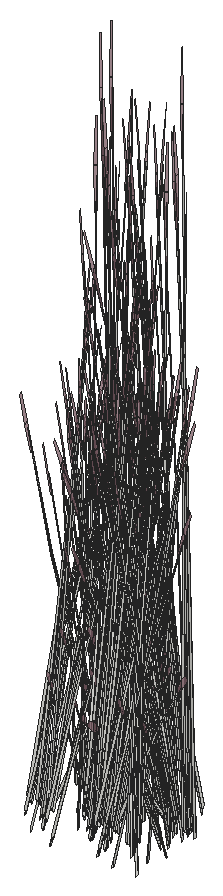
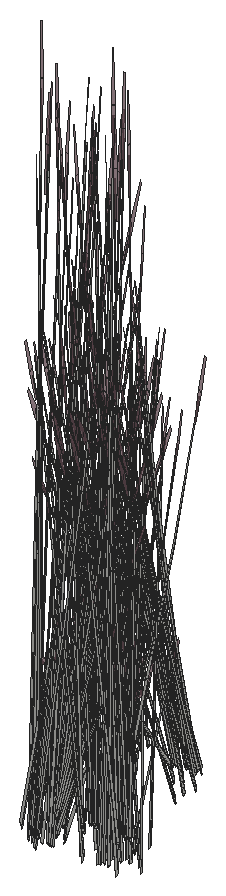
# SketchUp Ruby script. Lengths in inches.
U = 1.inch
M = Sketchup.active_model
def pt(a) = Geom::Point3d.new(a.map { |v| v * U })
def face(e, loops, mat)
  f = e.add_face(loops[0].map { |a| pt(a) })
  loops[1..].each { |l| e.add_face(l.map { |a| pt(a) }).erase! }
  f.material = f.back_material = mat if mat
  f
end
# faces: each face lists its corners as indices into pts; further lists are holes
def faces(e, pts, list, mat = nil) = list.each { |f| face(e, (f[0].is_a?(Array) ? f : [f]).map { |l| l.map { |i| pts[i] } }, mat) }
# xy, xz, yz: faces in a plane at the given z, y or x. An outline is a flat list of corners, or four numbers for a rectangle; further outlines are holes
def ring(l) = l.size == 4 ? [[l[0], l[1]], [l[2], l[1]], [l[2], l[3]], [l[0], l[3]]] : l.each_slice(2).to_a
def flat(e, list, mat, &to3) = list.each { |f| face(e, (f[0].is_a?(Array) ? f : [f]).map { |l| ring(l).map { |u, v| to3.(u, v) } }, mat) }
def xy(e, z, list, mat = nil) = flat(e, list, mat) { |x, y| [x, y, z] }
def xz(e, y, list, mat = nil) = flat(e, list, mat) { |x, z| [x, y, z] }
def yz(e, x, list, mat = nil) = flat(e, list, mat) { |y, z| [x, y, z] }
def lines(e, pts, list) = list.each { |a, b| e.add_line(pt(pts[a]), pt(pts[b])) }
# prism: a flat outline (further loops are holes) pulled along v
def prism(e, loops, v, mat = nil)
  f = face(e, loops, mat); d = Geom::Vector3d.new(v.map { |x| x * U })
  f.pushpull(f.normal.samedirection?(d) ? d.length : -d.length)
end
def box(e, o, s, mat = nil) = prism(e, [[o, [o[0] + s[0], o[1], o[2]], [o[0] + s[0], o[1] + s[1], o[2]], [o[0], o[1] + s[1], o[2]]]], [0, 0, s[2]], mat)
def at(x, y, z, deg = 0) = Geom::Transformation.translation(pt([x, y, z])) * Geom::Transformation.rotation(ORIGIN, Z_AXIS, deg.degrees)
def axes(o, x, y, z) = Geom::Transformation.new([*x, 0, *y, 0, *z, 0, *pt(o).to_a, 1])
def part(name) = M.definitions.add(name)
# library, detail: a bought-in or finely detailed component or shape, given as its bounding box
def library(name, o, s) = part(name).tap { |d| box(d.entities, o, s) }
def detail(e, o, s) = box(e.add_group.entities, o, s)
def put(e, d, t, mat = nil) = e.add_instance(d, t).tap { |i| i.material = mat if mat }
def group(e, t, mat = nil) = e.add_group.tap { |g| g.transformation = t; g.material = mat if mat }.entities
root = M.entities
M.materials.add("LightPink_Translucent").color = [144, 107, 117]
M.materials["LightPink_Translucent"].alpha = 0.75
c1 = part("blade")
p = [[2.15,0.21,22],[0,0.17,0],[0.09,0.45,0],[2.18,0.31,22],[2.29,0.31,22],[0.38,0.45,0],
  [2.48,0.24,33],[2.49,0.24,33],[2.48,0.22,33]]
faces(c1.entities,p,[[0,1,2,3],[4,5,2,3],[6,3,4,7],[8,0,3,6]])
c2 = part("seeds")
p = [[0.3,-0.1,1.38],[-0.01,-0.03,1.59],[-0.01,-0.03,0.03],[0.14,-0.07,-0.07],[0.29,-0.03,3],[0.15,0.01,3.11]]
faces(c2.entities,p,[[0,1,2,3],[1,0,4,5]],"LightPink_Translucent")
c3 = part("blade with seeds")
put(c3.entities,c1,at(0,0,0))
put(c3.entities,c2,axes([2.4,0.25,30.99],[1.5799,-0.05474,1.17369],[-0.12525,1.92788,0.29478],[-0.07173,-0.02425,1.56792]))
put(root,c3,axes([344.03,660.33,622.98],[-0.16845,-0.3792,-0.71045],[0.34676,-0.21133,0.08574],[-0.03939,-0.18322,1.00501]))
put(root,c3,axes([343.63,653.34,623.09],[0.00775,-0.24075,1.54345],[0.34877,0.12716,0.21329],[-0.03022,0.25658,0.72882]))
put(root,c3,axes([342.07,661.57,623.05],[-0.30722,0.06665,0.35414],[-0.08112,-0.381,-0.4572],[0.08804,-0.10234,0.87481]))
put(root,c3,axes([341.1875,660.5,621.875],[-0.06572,0.16029,1.71376],[-0.27569,-0.33172,0.13857],[0.12437,-0.20675,0.73262]))
put(root,c3,axes([344.1,660.38,623.05],[-0.1064,0.35863,0.35414],[-0.31043,-0.1046,-0.4572],[-0.02846,-0.14439,0.87481]))
put(root,c3,axes([342.53,653.1,624.6875],[0.16845,0.3792,-0.71045],[-0.34676,0.21133,0.08574],[0.03939,0.18322,1.00501]))
put(root,c3,axes([343.84,652.875,624.73],[0.25266,0.31335,-0.5672],[-0.2669,0.27442,-0.43934],[-0.03844,0.15921,1.08528]))
put(root,c3,axes([342.23,661.6,623.03],[-0.32648,-0.25715,-0.1216],[0.18809,-0.3724,-0.67495],[0.09224,-0.12945,1.02557]))
put(root,c3,axes([344.21,662.4,620.3],[-0.32829,-0.4014,-0.06131],[0.32849,-0.40164,0],[-0.01146,-0.01402,1.75571]))
put(root,c3,axes([341.71,660.51,620.375],[0.22066,-0.46731,0],[0.36918,0.26061,-0.51607],[0.08408,0.05936,1.63711]))
put(root,c3,axes([342.08,660.31,619.49],[-0.05283,-0.03674,1.76342],[-0.13569,-0.41045,-0.26939],[0.09154,-0.11138,0.30037]))
put(root,c3,axes([343.57,652.71,625.12],[0.3879,0.02311,-0.13498],[-0.0106,0.43749,-0.74919],[-0.02694,0.1685,1.13838]))
put(root,c3,axes([343.56,653.34,622.55],[0.32063,-0.08258,0.06507],[0.07371,0.33271,-0.86304],[-0.02033,0.16842,0.7736]))
put(root,c3,axes([343.74,659.48,619.49],[-0.0592,0.0168,1.76342],[-0.32738,-0.18913,-0.26939],[0.00549,-0.15776,0.30037]))
put(root,c3,axes([342.66,653.18,624.39],[0.34695,0.11691,-0.51099],[-0.11892,0.40083,-0.3958],[0.03181,0.16138,0.97773]))
put(root,c3,axes([342.36,653.2,624.74],[0.34538,-0.21713,-0.1216],[0.16972,0.38536,-0.67495],[0.04557,0.16239,1.02557]))
put(root,c3,axes([344.07,660,622.53],[0.1064,-0.35863,-0.35414],[0.31043,0.1046,0.4572],[-0.02846,-0.14439,0.87481]))
put(root,c3,axes([344.125,652.42,623.6],[-0.00864,-0.17899,1.71376],[0.37441,0.11874,0.13857],[-0.02316,0.25508,0.73262]))
put(root,c3,axes([343.55,661.94,620.36],[0.15345,0.52148,0.45755],[-0.43845,0.18134,0.17955],[0.00536,-0.09582,1.58856]))
put(root,c3,axes([342.07,661.3,622.68],[-0.09067,-0.42583,-0.51099],[0.34336,-0.07449,-0.3958],[0.0984,-0.11438,0.97773]))
put(root,c3,axes([343.48,661.875,620.21],[0.17124,-0.42022,-0.44739],[0.35581,0.20224,0.21531],[0,-0.09687,1.43643]))
put(root,c3,axes([342.99,661.97,620.26],[-0.21881,-0.29821,-0.06488],[0.23965,-0.27324,-0.29416],[0.0679,-0.01924,0.97024]))
put(root,c3,axes([342.49,660.45,620.77],[-0.11756,0.2374,1.1486],[-0.10105,-0.31895,0.84392],[0.09709,-0.07992,0.25299]))
put(root,c3,axes([342.35,661.51,622.73],[0.2423,0.19613,0.0643],[-0.14107,0.2793,0.50621],[0.07768,-0.0903,0.77189]))
put(root,c3,axes([344.2,660.06,622.73],[0.26007,-0.1585,0.0643],[0.12729,0.28902,0.50621],[-0.02512,-0.1274,0.77189]))
put(root,c3,axes([342.28,661.42,622.73],[0.08753,0.42921,0.48003],[-0.34336,0.07449,0.3958],[0.1012,-0.10094,0.9933]))
put(root,c3,axes([344.1,661.98,620.21],[0,-0.53961,0],[0.44133,0,0],[0,0,1.79456]))
put(root,c3,axes([344.11,660.09,622.73],[0.34777,0.12192,0.48003],[-0.11892,0.40083,0.3958],[-0.0209,-0.15763,0.9933]))
put(root,c3,axes([343.6875,662.08,620.43],[0.39767,0.22603,0.24065],[-0.19139,0.46966,0.50002],[0,-0.10827,1.60543]))
put(root,c3,axes([343.56,661.77,620.72],[-0.38326,0.02879,0.44739],[-0.03466,-0.47788,-0.21531],[0.06861,-0.04843,1.43643]))
put(root,c3,axes([344.39,653.34,624.79],[-0.34777,-0.12192,0.53283],[0.11892,-0.40083,0.43934],[0.0209,0.15763,1.10256]))
put(root,c3,axes([343.03,661.49,622.71],[-0.0461,-0.00354,1.77383],[-0.19143,-0.37951,-0.16761],[0.07688,-0.12478,0.31391]))
put(root,c3,axes([342.85,652.35,623.58],[-0.08068,-0.14973,1.71376],[0.3728,-0.12606,0.13857],[0.08426,0.23506,0.73262]))
put(root,c3,axes([344.3,653.37,624.46],[-0.26007,0.1585,0.0643],[-0.12729,-0.28902,0.50621],[0.02512,0.1274,0.77189]))
put(root,c3,axes([342.32,661.34,622.53],[0.30722,-0.06665,-0.35414],[0.08112,0.381,0.4572],[0.08804,-0.10234,0.87481]))
put(root,c3,axes([342.08,661.47,622.98],[0.18436,-0.36797,-0.71045],[0.32306,0.26151,0.08574],[0.11008,-0.13332,1.00501]))
put(root,c3,axes([342.24,662.6,623.03],[-0.17758,-0.42229,-0.1216],[0.31518,-0.20752,-0.67495],[0.13282,-0.05572,1.02557]))
put(root,c3,axes([343.2,660.375,620.375],[-0.22066,-0.46731,0],[0.36918,-0.26061,-0.51607],[0.08408,-0.05936,1.63711]))
put(root,c3,axes([344.125,659.25,620.77],[0.04528,0.27194,1.1486],[-0.25117,-0.15062,0.84392],[0.02703,-0.13924,0.25299]))
put(root,c3,axes([343.89,661.64,620.36],[-0.29264,0.42323,0.45755],[-0.34767,-0.3736,0.17955],[0.07055,-0.04224,1.58856]))
put(root,c3,axes([344.35,653.28,621.22],[0.05712,-0.02538,1.76342],[0.34359,0.13968,-0.26939],[0.01005,0.15742,0.30037]))
put(root,c3,axes([344.43,653.42,624.25],[-0.1064,0.35863,-0.35414],[-0.31043,-0.1046,0.4572],[0.02846,0.14439,0.87481]))
put(root,c3,axes([342.23,662.24,622.68],[0.09562,-0.42421,-0.51099],[0.32782,0.1454,-0.3958],[0.13199,-0.0389,0.97773]))
put(root,c3,axes([345.2,659.69,622.71],[-0.03584,0.03562,1.77383],[-0.35118,-0.12018,-0.16761],[-0.01271,-0.15545,0.31391]))
put(root,c3,axes([344.92,660.72,623.03],[-0.3879,-0.02311,-0.1216],[0.0106,-0.43749,-0.67495],[0.02694,-0.1685,1.02557]))
put(root,c3,axes([343.17,652.65,622.3],[0.00623,-0.15459,1.43002],[0.29764,-0.17268,-0.30754],[0.09188,0.18503,0.61141]))
put(root,c3,axes([342.34,661.13,620.59],[-0.12609,-0.01381,1.43002],[-0.12917,-0.37055,-0.30754],[0.1549,-0.10482,0.61141]))
put(root,c3,axes([348.55,661.52,621.875],[0.14639,-0.01056,1.71376],[-0.09712,0.45778,0.13857],[-0.20862,-0.02831,0.73262]))
put(root,c3,axes([344.77,660.79,623.05],[-0.23881,0.24554,0.35414],[-0.22606,-0.28036,-0.4572],[0.0344,-0.14245,0.87481]))
put(root,c3,axes([344.21,654.06,624.44],[0.04474,0.0751,1.74944],[0.36104,0.0295,-0.27667],[0.03631,0.16562,0.14031]))
put(root,c3,axes([343.63,661.67,620.67],[-0.04113,-0.53214,-0.29095],[0.42835,-0.03218,-0.50002],[0.07543,-0.07088,1.59708]))
put(root,c3,axes([344.66,660.55,622.68],[-0.25266,-0.31335,-0.51099],[0.2669,-0.27442,-0.3958],[0.03844,-0.15921,0.97773]))
put(root,c3,axes([342.58,662.36,619.98],[-0.22732,0.05597,1.41583],[-0.03618,-0.44548,0.08104],[0.15921,-0.06743,0.80566]))
put(root,c3,axes([343.58,660.49,620.03],[0.32928,0.11539,-0.30978],[-0.08291,0.40636,0.30978],[0.06638,-0.04686,1.38974]))
put(root,c3,axes([344.49,660,620.59],[-0.10032,0.0944,1.43002],[-0.30046,-0.16522,-0.30754],[0.05569,-0.20547,0.61141]))
put(root,c3,axes([344.46,653.1,624.71],[0.16845,0.3792,-0.71045],[-0.34676,0.21133,0.08574],[0.03939,0.18322,1.00501]))
put(root,c3,axes([342.17,662.4,622.98],[0.31014,-0.20596,-0.71045],[0.17284,0.42397,0.08574],[0.14985,-0.04816,1.00501]))
put(root,c3,axes([343.5,660.3,620.02],[0.33032,-0.23318,-0.49651],[0.19744,0.41812,0],[0.07523,-0.05311,1.57504]))
put(root,c3,axes([343.21,661.94,622.72],[0.04898,-0.07104,1.74944],[-0.06269,-0.43574,-0.27667],[0.12289,-0.08262,0.14031]))
put(root,c3,axes([347.64,652.27,624.1],[0.06572,-0.16029,1.71376],[0.27569,0.33172,0.13857],[-0.12437,0.20675,0.73262]))
put(root,c3,axes([344.63,660.74,620.48],[-0.33032,-0.23318,0.49651],[0.19744,-0.41812,0],[0.07523,0.05311,1.57504]))
put(root,c3,axes([344.74,660.7,622.98],[0.00918,-0.43138,-0.71045],[0.38672,0.02897,0.08574],[0.04081,-0.18275,1.00501]))
put(root,c3,axes([344.59,653.18,624.41],[0.34695,0.11691,-0.51099],[-0.11892,0.40083,-0.3958],[0.03181,0.16138,0.97773]))
put(root,c3,axes([344.29,653.2,624.76],[0.34538,-0.21713,-0.1216],[0.16972,0.38536,-0.67495],[0.04557,0.16239,1.02557]))
put(root,c3,axes([346.89,653.1,624.94],[-0.00877,0.09229,1.74944],[0.24897,0.32105,-0.27667],[-0.06518,0.15182,0.14031]))
put(root,c3,axes([348.99,661.09,622.98],[-0.35281,-0.01123,-0.71045],[0.0237,-0.47284,0.08574],[-0.14947,-0.0499,1.00501]))
put(root,c3,axes([348.7,661.21,620.59],[0.06891,0.12984,1.43002],[-0.15879,0.35293,-0.30754],[-0.16304,-0.08436,0.61141]))
put(root,c3,axes([348.83,660.78,621.875],[0.1311,0.08035,1.71376],[-0.27131,0.33708,0.13857],[-0.16909,-0.15206,0.73262]))
put(root,c3,axes([344.9,660.4375,622.53],[0.23881,-0.24554,-0.35414],[0.22606,0.28036,0.4572],[0.0344,-0.14245,0.87481]))
put(root,c3,axes([344.99,660.5625,622.73],[0.29004,0.02173,0.0643],[-0.00795,0.32812,0.50621],[0.03035,-0.12569,0.77189]))
put(root,c3,axes([345.28,660.02,622.72],[-0.00341,-0.09282,1.74944],[-0.28775,-0.26825,-0.27667],[0.04449,-0.16261,0.14031]))
put(root,c3,axes([343.89,661.26,620.06],[0.23773,-0.35053,-0.62353],[0.29532,0.31785,-0.16365],[0.09526,-0.08744,1.37633]))
put(root,c3,axes([344.89,660.53,622.73],[0.25132,0.3182,0.48003],[-0.2669,0.27442,0.3958],[0.04636,-0.14929,0.9933]))
put(root,c3,axes([348.87,661.1875,622.68],[-0.25628,0.30892,-0.51099],[-0.22444,-0.32634,-0.3958],[-0.13021,-0.047,0.97773]))
put(root,c3,axes([348.51,660.32,622.71],[0.02617,0.04654,1.77383],[-0.12614,0.41836,-0.16761],[-0.12775,0.00303,0.31391]))
put(root,c3,axes([344.78,652.35,623.6],[-0.08068,-0.14973,1.71376],[0.3728,-0.12606,0.13857],[0.08426,0.23506,0.73262]))
put(root,c3,axes([348.8,660.04,622.72],[-0.07594,-0.00329,1.74944],[-0.24177,0.32918,-0.27667],[-0.129,-0.06726,0.14031]))
put(root,c3,axes([345.1875,661.54,623.05],[-0.30722,0.06665,0.35414],[-0.08112,-0.381,-0.4572],[0.08804,-0.10234,0.87481]))
put(root,c3,axes([347.6,653.88,622.82],[0.11138,-0.07357,1.43002],[0.27499,0.22183,-0.30754],[-0.08185,0.19194,0.61141]))
put(root,c3,axes([344.3,660.48,621.875],[-0.06572,0.16029,1.71376],[-0.27569,-0.33172,0.13857],[0.12437,-0.20675,0.73262]))
put(root,c3,axes([349,660.86,623.03],[-0.0189,0.47427,-0.1216],[-0.35781,-0.01296,-0.67495],[-0.13781,-0.03295,1.02557]))
put(root,c3,axes([348.77,660.9,622.53],[-0.20082,-0.29199,-0.35414],[0.2293,-0.2764,0.4572],[-0.1165,-0.04206,0.87481]))
put(root,c3,axes([348.29,661.6,620.77],[0.22533,-0.03337,1.1486],[-0.14293,0.29403,0.84392],[-0.11135,-0.04411,0.25299]))
put(root,c3,axes([345.34,661.58,623.03],[-0.32648,-0.25715,-0.1216],[0.18809,-0.3724,-0.67495],[0.09224,-0.12945,1.02557]))
put(root,c3,axes([347.72,653.17,624.75],[-0.23881,0.24554,-0.35414],[-0.22606,-0.28036,0.4572],[-0.0344,0.14245,0.87481]))
put(root,c3,axes([348.83,652.5,623.57],[0.06572,-0.16029,1.71376],[0.27569,0.33172,0.13857],[-0.12437,0.20675,0.73262]))
put(root,c3,axes([348.74,660.79,623.09],[0.29147,-0.34417,0.53763],[0.25138,0.3655,0.4433],[-0.13675,-0.06349,1.11249]))
put(root,c3,axes([344.82,660.49,620.375],[0.22066,-0.46731,0],[0.36918,0.26061,-0.51607],[0.08408,0.05936,1.63711]))
put(root,c3,axes([345.19,660.29,619.49],[-0.05283,-0.03674,1.76342],[-0.13569,-0.41045,-0.26939],[0.09154,-0.11138,0.30037]))
put(root,c3,axes([345.1,652.65,622.32],[0.00623,-0.15459,1.43002],[0.29764,-0.17268,-0.30754],[0.09188,0.18503,0.61141]))
put(root,c3,axes([346.87,654.04,624.93],[0.04004,-0.02816,1.77383],[0.33095,0.18728,-0.16761],[-0.00778,0.15594,0.31391]))
put(root,c3,axes([345.18,661.27,622.68],[-0.09067,-0.42583,-0.51099],[0.34336,-0.07449,-0.3958],[0.0984,-0.11438,0.97773]))
put(root,c3,axes([348.09,653.33,624.41],[-0.00877,0.09229,1.74944],[0.24897,0.32105,-0.27667],[-0.06518,0.15182,0.14031]))
put(root,c3,axes([347.875,652.91,625.5625],[-0.00918,0.43138,-0.7886],[-0.38672,-0.02897,0.09517],[-0.04081,0.18275,1.11556]))
put(root,c3,axes([346.11,661.95,620.26],[-0.21881,-0.29821,-0.06488],[0.23965,-0.27324,-0.29416],[0.0679,-0.01924,0.97024]))
put(root,c3,axes([347.87,654.125,622.99],[-0.00913,-0.2773,1.1486],[0.22824,0.19778,0.84392],[-0.04489,0.13217,0.25299]))
put(root,c3,axes([348.88,660.78,622.73],[0.01777,-0.35463,0.0643],[0.26836,0.00972,0.50621],[-0.1028,-0.03711,0.77189]))
put(root,c3,axes([349.64,662.74,620.06],[-0.36714,-0.07646,-0.62353],[0.07747,-0.47163,-0.16365],[-0.10956,-0.05715,1.37633]))
put(root,c3,axes([349.7,660.17,623.43],[-0.23555,0.44708,-0.13619],[-0.34112,-0.25757,-0.75594],[-0.11858,-0.12631,1.14864]))
put(root,c3,axes([345.6,660.43,620.77],[-0.11756,0.2374,1.1486],[-0.10105,-0.31895,0.84392],[0.09709,-0.07992,0.25299]))
put(root,c3,axes([345.46,661.48,622.73],[0.2423,0.19613,0.0643],[-0.14107,0.2793,0.50621],[0.07768,-0.0903,0.77189]))
put(root,c3,axes([349.06,661.05,623.05],[0.20082,0.29199,0.35414],[-0.2293,0.2764,-0.4572],[-0.1165,-0.04206,0.87481]))
put(root,c3,axes([349.6,660.53,622.98],[-0.30095,-0.22541,-0.71045],[0.21388,-0.395,0.08574],[-0.10904,-0.13459,1.00501]))
put(root,c3,axes([349.46,660.54,622.68],[-0.34827,0.11086,-0.51099],[-0.06092,-0.41983,-0.3958],[-0.09354,-0.12031,0.97773]))
put(root,c3,axes([347.75,653.52,623.59],[0.00775,-0.24075,1.54345],[0.34877,0.12716,0.21329],[-0.03022,0.25658,0.72882]))
put(root,c3,axes([345.4,661.4,622.73],[0.08753,0.42921,0.48003],[-0.34336,0.07449,0.3958],[0.1012,-0.10094,0.9933]))
put(root,c3,axes([349.01,660.16,619.49],[-0.03419,0.06144,1.76342],[-0.3455,0.13246,-0.26939],[-0.08346,-0.12049,0.30037]))
put(root,c3,axes([346.15,661.47,622.71],[-0.0461,-0.00354,1.77383],[-0.19143,-0.37951,-0.16761],[0.07688,-0.12478,0.31391]))
put(root,c3,axes([345.4375,661.32,622.53],[0.30722,-0.06665,-0.35414],[0.08112,0.381,0.4572],[0.08804,-0.10234,0.87481]))
put(root,c3,axes([345.19,661.45,622.98],[0.18436,-0.36797,-0.71045],[0.32306,0.26151,0.08574],[0.11008,-0.13332,1.00501]))
put(root,c3,axes([348.8,654.11,622.28],[0.11138,-0.07357,1.43002],[0.27499,0.22183,-0.30754],[-0.08185,0.19194,0.61141]))
put(root,c3,axes([347.95,653.05,625.23],[0.25266,0.31335,-0.5672],[-0.2669,0.27442,-0.43934],[-0.03844,0.15921,1.08528]))
put(root,c3,axes([345.36,662.58,623.03],[-0.17758,-0.42229,-0.1216],[0.31518,-0.20752,-0.67495],[0.13282,-0.05572,1.02557]))
put(root,c3,axes([348.8,660.4,620.13],[-0.10181,0.3808,-0.03893],[-0.31336,-0.11714,-0.17649],[-0.04758,-0.06228,0.58215]))
put(root,c3,axes([347.6875,652.89,625.62],[0.3879,0.02311,-0.13498],[-0.0106,0.43749,-0.74919],[-0.02694,0.1685,1.13838]))
put(root,c3,axes([347.68,653.52,623.05],[0.32063,-0.08258,0.06507],[0.07371,0.33271,-0.86304],[-0.02033,0.16842,0.7736]))
put(root,c3,axes([349.61,659.11,622.71],[-0.00658,0.0559,1.77383],[-0.32474,0.20287,-0.16761],[-0.09556,-0.1037,0.31391]))
put(root,c3,axes([349.26,659.92,620.59],[-0.02137,0.15256,1.43002],[-0.31245,0.12771,-0.30754],[-0.07303,-0.19719,0.61141]))
put(root,c3,axes([349.37,660.3125,621.875],[0.08068,0.14973,1.71376],[-0.3728,0.12606,0.13857],[-0.08426,-0.23506,0.73262]))
put(root,c3,axes([348.24,652.6,624.1],[-0.00864,-0.17899,1.71376],[0.37441,0.11874,0.13857],[-0.02316,0.25508,0.73262]))
put(root,c3,axes([348.91,653.41,624.22],[-0.23881,0.24554,-0.35414],[-0.22606,-0.28036,0.4572],[-0.0344,0.14245,0.87481]))
put(root,c3,axes([345.34,662.22,622.68],[0.09562,-0.42421,-0.51099],[0.32782,0.1454,-0.3958],[0.13199,-0.0389,0.97773]))
put(root,c3,axes([349.5,660.23,622.53],[-0.05451,-0.37564,-0.35414],[0.31161,-0.09919,0.4572],[-0.0837,-0.10765,0.87481]))
put(root,c3,axes([348.625,662.14,620.375],[-0.44133,0,0],[0,-0.52122,-0.51607],[0,-0.11871,1.63711]))
put(root,c3,axes([348.06,654.28,624.4],[0.04004,-0.02816,1.77383],[0.33095,0.18728,-0.16761],[-0.00778,0.15594,0.31391]))
put(root,c3,axes([345.46,661.11,620.59],[-0.12609,-0.01381,1.43002],[-0.12917,-0.37055,-0.30754],[0.1549,-0.10482,0.61141]))
put(root,c3,axes([349.68,660.54,623.05],[0.05451,0.37564,0.35414],[-0.31161,0.09919,-0.4572],[-0.0837,-0.10765,0.87481]))
put(root,c3,axes([348.97,662,620.33],[-0.32829,0.39208,0.30756],[-0.32849,-0.38796,-0.36492],[-0.01146,-0.11134,1.64885]))
put(root,c3,axes([349.07,653.15,625.03],[-0.00918,0.43138,-0.7886],[-0.38672,-0.02897,0.09517],[-0.04081,0.18275,1.11556]))
put(root,c3,axes([345.69,662.34,619.98],[-0.22732,0.05597,1.41583],[-0.03618,-0.44548,0.08104],[0.15921,-0.06743,0.80566]))
put(root,c3,axes([350.32,663.08,621.33],[0.305,0.18805,1.51261],[-0.29879,0.40513,0.59816],[-0.13384,-0.24012,1.26806]))
put(root,c3,axes([349.0625,654.36,622.46],[-0.00913,-0.2773,1.1486],[0.22824,0.19778,0.84392],[-0.04489,0.13217,0.25299]))
put(root,c3,axes([349.16,659.67,620.77],[0.18411,0.16231,1.1486],[-0.26813,0.09757,0.84392],[-0.05737,-0.12474,0.25299]))
put(root,c3,axes([349.83,662.59,620.21],[-0.21202,-0.39143,-0.44739],[0.32115,-0.27564,0.21531],[-0.06861,-0.04843,1.43643]))
put(root,c3,axes([348.51,653.52,625.29],[-0.34777,-0.12192,0.53283],[0.11892,-0.40083,0.43934],[0.0209,0.15763,1.10256]))
put(root,c3,axes([349.54,660.1,623.09],[0.39316,-0.11987,0.53763],[0.06823,0.47021,0.4433],[-0.09247,-0.13858,1.11249]))
put(root,c3,axes([348.41,653.55,624.96],[-0.26007,0.1585,0.0643],[-0.12729,-0.28902,0.50621],[0.02512,0.1274,0.77189]))
put(root,c3,axes([348.94,653.75,623.05],[0.00775,-0.24075,1.54345],[0.34877,0.12716,0.21329],[-0.03022,0.25658,0.72882]))
put(root,c3,axes([345.28,662.375,622.98],[0.31014,-0.20596,-0.71045],[0.17284,0.42397,0.08574],[0.14985,-0.04816,1.00501]))
put(root,c3,axes([349.63,660.2,622.73],[0.16041,-0.29625,0.0643],[0.22843,0.17248,0.50621],[-0.07385,-0.09498,0.77189]))
put(root,c3,axes([346.32,661.92,622.72],[0.04898,-0.07104,1.74944],[-0.06269,-0.43574,-0.27667],[0.12289,-0.08262,0.14031]))
put(root,c3,axes([349.86,662.82,620.4375],[0.09355,-0.55261,-0.23429],[0.44354,0.09633,0.51271],[-0.0775,-0.07631,1.5644]))
put(root,c3,axes([349.15,653.29,624.7],[0.25266,0.31335,-0.5672],[-0.2669,0.27442,-0.43934],[-0.03844,0.15921,1.08528]))
put(root,c3,axes([349.98,659.32,622.72],[-0.05398,-0.06539,1.74944],[-0.36026,0.04145,-0.27667],[-0.0575,-0.15639,0.14031]))
put(root,c3,axes([348.47,653.46,621.72],[0.05712,-0.02538,1.76342],[0.34359,0.13968,-0.26939],[0.01005,0.15742,0.30037]))
put(root,c3,axes([348.73,661.78,620.02],[0,-0.46636,-0.49651],[0.39487,0,0],[0,-0.10622,1.57504]))
put(root,c3,axes([348.89,662.22,620.48],[0,0.46636,0.49651],[-0.39487,0,0],[0,-0.10622,1.57504]))
put(root,c3,axes([348.55,653.6,624.75],[-0.1064,0.35863,-0.35414],[-0.31043,-0.1046,0.4572],[0.02846,0.14439,0.87481]))
put(root,c3,axes([348.88,653.125,625.09],[0.3879,0.02311,-0.13498],[-0.0106,0.43749,-0.74919],[-0.02694,0.1685,1.13838]))
put(root,c3,axes([348.875,653.76,622.51],[0.32063,-0.08258,0.06507],[0.07371,0.33271,-0.86304],[-0.02033,0.16842,0.7736]))
put(root,c3,axes([349.76,662.32,620.67],[-0.39748,-0.22252,-0.29095],[0.19139,-0.46966,-0.50002],[-0.01249,-0.11531,1.59708]))
put(root,c3,axes([349.44,652.84,623.57],[-0.00864,-0.17899,1.71376],[0.37441,0.11874,0.13857],[-0.02316,0.25508,0.73262]))
put(root,c3,axes([348.33,654.24,624.94],[0.04474,0.0751,1.74944],[0.36104,0.0295,-0.27667],[0.03631,0.16562,0.14031]))
put(root,c3,axes([349.58,661.85,620.1],[-0.14494,-0.47823,-0.69835],[0.41752,-0.17223,-0.18329],[-0.01602,-0.16194,1.54149]))
put(root,c3,axes([350.53,660.33,623.03],[-0.34538,0.21713,-0.1216],[-0.16972,-0.38536,-0.67495],[-0.04557,-0.16239,1.02557]))
put(root,c3,axes([350.23,660.35,622.68],[-0.34695,-0.11691,-0.51099],[0.11892,-0.40083,-0.3958],[-0.03181,-0.16138,0.97773]))
put(root,c3,axes([348.89,661.79,620.03],[0.24637,-0.29097,-0.30978],[0.24637,0.29097,0.30978],[0,-0.09372,1.38974]))
put(root,c3,axes([350.01,659.91,620.13],[-0.2439,0.26754,-0.03893],[-0.22348,-0.29302,-0.17649],[-0.01573,-0.08303,0.58215]))
put(root,c3,axes([351.92,652.96,623.01],[0.08815,-0.14329,1.71376],[0.22258,0.38678,0.13857],[-0.15267,0.17614,0.73262]))
put(root,c3,axes([351.22,654.47,620.63],[0.04734,0.04659,1.76342],[0.08027,0.4317,-0.26939],[-0.10492,0.09206,0.30037]))
put(root,c3,axes([348.58,653.28,625.21],[0.16845,0.3792,-0.71045],[-0.34676,0.21133,0.08574],[0.03939,0.18322,1.00501]))
put(root,c3,axes([349.79,662.45,620.72],[-0.17124,0.42022,0.44739],[-0.35581,-0.20224,-0.21531],[0,-0.09687,1.43643]))
put(root,c3,axes([350.36,660.43,622.98],[-0.16845,-0.3792,-0.71045],[0.34676,-0.21133,0.08574],[-0.03939,-0.18322,1.00501]))
put(root,c3,axes([349.7,653.76,624.75],[-0.34777,-0.12192,0.53283],[0.11892,-0.40083,0.43934],[0.0209,0.15763,1.10256]))
put(root,c3,axes([349.61,653.79,624.42],[-0.26007,0.1585,0.0643],[-0.12729,-0.28902,0.50621],[0.02512,0.1274,0.77189]))
put(root,c3,axes([350.43,660.48,623.05],[-0.1064,0.35863,0.35414],[-0.31043,-0.1046,-0.4572],[-0.02846,-0.14439,0.87481]))
put(root,c3,axes([351.85,653.32,623.01],[0.06572,-0.16029,1.71376],[0.27569,0.33172,0.13857],[-0.12437,0.20675,0.73262]))
put(root,c3,axes([348.7,653.36,624.91],[0.34695,0.11691,-0.51099],[-0.11892,0.40083,-0.3958],[0.03181,0.16138,0.97773]))
put(root,c3,axes([348.41,653.375,625.26],[0.34538,-0.21713,-0.1216],[0.16972,0.38536,-0.67495],[0.04557,0.16239,1.02557]))
put(root,c3,axes([351.64,653.38,623.82],[0.09067,0.42583,-0.51099],[-0.34336,0.07449,-0.3958],[-0.0984,0.11438,0.97773]))
put(root,c3,axes([351.1,654.15,623.85],[-0.00877,0.09229,1.74944],[0.24897,0.32105,-0.27667],[-0.06518,0.15182,0.14031]))
put(root,c3,axes([349.66,653.7,621.18],[0.05712,-0.02538,1.76342],[0.34359,0.13968,-0.26939],[0.01005,0.15742,0.30037]))
put(root,c3,axes([350.07,659.58,619.49],[-0.0592,0.0168,1.76342],[-0.32738,-0.18913,-0.26939],[0.00549,-0.15776,0.30037]))
put(root,c3,axes([349.74,653.84,624.22],[-0.1064,0.35863,-0.35414],[-0.31043,-0.1046,0.4572],[0.02846,0.14439,0.87481]))
put(root,c3,axes([350.39,660.1,622.53],[0.1064,-0.35863,-0.35414],[0.31043,0.1046,0.4572],[-0.02846,-0.14439,0.87481]))
put(root,c3,axes([349.87,662.04,620.36],[0.15345,0.52148,0.45755],[-0.43845,0.18134,0.17955],[0.00536,-0.09582,1.58856]))
put(root,c3,axes([349.8,661.97,620.21],[0.17124,-0.42022,-0.44739],[0.35581,0.20224,0.21531],[0,-0.09687,1.43643]))
put(root,c3,axes([351.48,653.08,624.17],[0.32648,0.25715,-0.1216],[-0.18809,0.3724,-0.67495],[-0.09224,0.12945,1.02557]))
put(root,c3,axes([349.52,654.48,624.41],[0.04474,0.0751,1.74944],[0.36104,0.0295,-0.27667],[0.03631,0.16562,0.14031]))
put(root,c3,axes([348.9,652.53,624.1],[-0.08068,-0.14973,1.71376],[0.3728,-0.12606,0.13857],[0.08426,0.23506,0.73262]))
put(root,c3,axes([350.52,660.16,622.73],[0.26007,-0.1585,0.0643],[0.12729,0.28902,0.50621],[-0.02512,-0.1274,0.77189]))
put(root,c3,axes([350.42,662.08,620.21],[0,-0.53961,0],[0.44133,0,0],[0,0,1.79456]))
put(root,c3,axes([350.43,660.1875,622.73],[0.34777,0.12192,0.48003],[-0.11892,0.40083,0.3958],[-0.0209,-0.15763,0.9933]))
put(root,c3,axes([350.01,662.18,620.43],[0.39767,0.22603,0.24065],[-0.19139,0.46966,0.50002],[0,-0.10827,1.60543]))
put(root,c3,axes([351.8125,654.93,621.73],[0.11138,-0.07357,1.43002],[0.27499,0.22183,-0.30754],[-0.08185,0.19194,0.61141]))
put(root,c3,axes([349.88,661.87,620.72],[-0.38326,0.02879,0.44739],[-0.03466,-0.47788,-0.21531],[0.06861,-0.04843,1.43643]))
put(root,c3,axes([349.77,653.52,624.67],[0.16845,0.3792,-0.71045],[-0.34676,0.21133,0.08574],[0.03939,0.18322,1.00501]))
put(root,c3,axes([351.93,654.125,623.87],[-0.25132,-0.3182,0.48003],[0.2669,-0.27442,0.3958],[-0.04636,0.14929,0.9933]))
put(root,c3,axes([349.52,660.47,620.375],[-0.22066,-0.46731,0],[0.36918,-0.26061,-0.51607],[0.08408,-0.05936,1.63711]))
put(root,c3,axes([350.12,654.74,625.34],[0.2439,-0.26754,-0.06488],[0.22348,0.29302,-0.29416],[0.01573,0.08303,0.97024]))
put(root,c3,axes([351.83,654.09,623.87],[-0.29004,-0.02173,0.0643],[0.00795,-0.32812,0.50621],[-0.03035,0.12569,0.77189]))
put(root,c3,axes([351.93,654.22,623.66],[-0.23881,0.24554,-0.35414],[-0.22606,-0.28036,0.4572],[-0.0344,0.14245,0.87481]))
put(root,c3,axes([349.9,653.59,624.37],[0.34695,0.11691,-0.51099],[-0.11892,0.40083,-0.3958],[0.03181,0.16138,0.97773]))
put(root,c3,axes([350.45,659.35,620.77],[0.04528,0.27194,1.1486],[-0.25117,-0.15062,0.84392],[0.02703,-0.13924,0.25299]))
put(root,c3,axes([349.22,652.83,622.82],[0.00623,-0.15459,1.43002],[0.29764,-0.17268,-0.30754],[0.09188,0.18503,0.61141]))
put(root,c3,axes([349.6,653.61,624.73],[0.34538,-0.21713,-0.1216],[0.16972,0.38536,-0.67495],[0.04557,0.16239,1.02557]))
